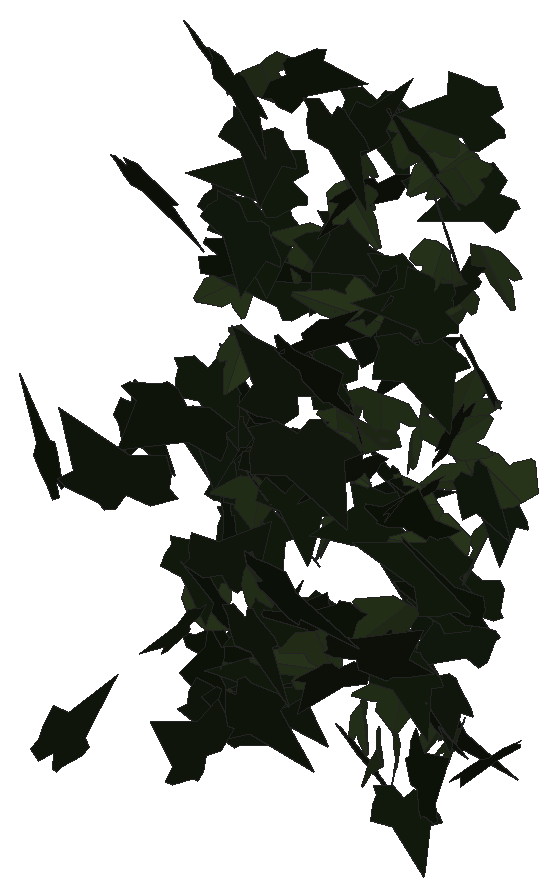
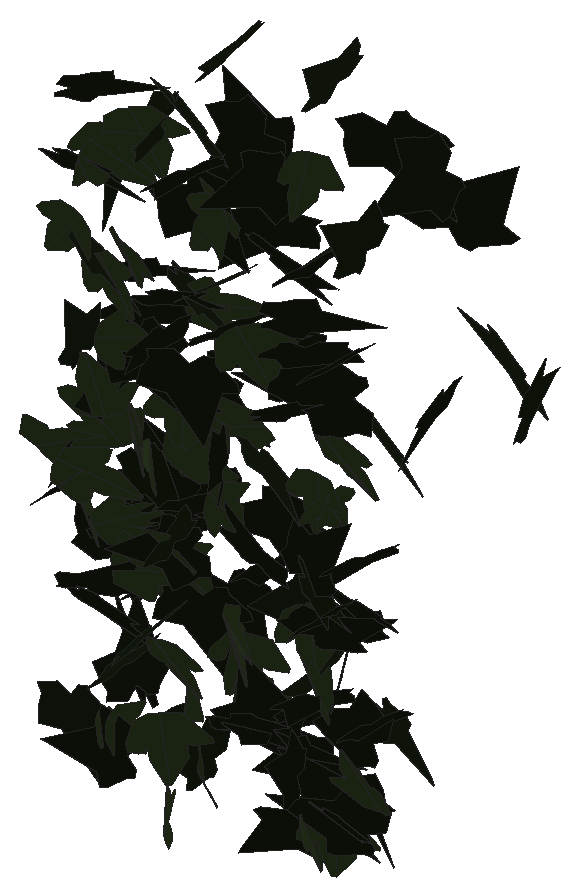
# SketchUp Ruby script. Lengths in inches.
U = 1.inch
M = Sketchup.active_model
def pt(a) = Geom::Point3d.new(a.map { |v| v * U })
def face(e, loops, mat)
  f = e.add_face(loops[0].map { |a| pt(a) })
  loops[1..].each { |l| e.add_face(l.map { |a| pt(a) }).erase! }
  f.material = f.back_material = mat if mat
  f
end
# faces: each face lists its corners as indices into pts; further lists are holes
def faces(e, pts, list, mat = nil) = list.each { |f| face(e, (f[0].is_a?(Array) ? f : [f]).map { |l| l.map { |i| pts[i] } }, mat) }
# xy, xz, yz: faces in a plane at the given z, y or x. An outline is a flat list of corners, or four numbers for a rectangle; further outlines are holes
def ring(l) = l.size == 4 ? [[l[0], l[1]], [l[2], l[1]], [l[2], l[3]], [l[0], l[3]]] : l.each_slice(2).to_a
def flat(e, list, mat, &to3) = list.each { |f| face(e, (f[0].is_a?(Array) ? f : [f]).map { |l| ring(l).map { |u, v| to3.(u, v) } }, mat) }
def xy(e, z, list, mat = nil) = flat(e, list, mat) { |x, y| [x, y, z] }
def xz(e, y, list, mat = nil) = flat(e, list, mat) { |x, z| [x, y, z] }
def yz(e, x, list, mat = nil) = flat(e, list, mat) { |y, z| [x, y, z] }
def lines(e, pts, list) = list.each { |a, b| e.add_line(pt(pts[a]), pt(pts[b])) }
# prism: a flat outline (further loops are holes) pulled along v
def prism(e, loops, v, mat = nil)
  f = face(e, loops, mat); d = Geom::Vector3d.new(v.map { |x| x * U })
  f.pushpull(f.normal.samedirection?(d) ? d.length : -d.length)
end
def box(e, o, s, mat = nil) = prism(e, [[o, [o[0] + s[0], o[1], o[2]], [o[0] + s[0], o[1] + s[1], o[2]], [o[0], o[1] + s[1], o[2]]]], [0, 0, s[2]], mat)
def at(x, y, z, deg = 0) = Geom::Transformation.translation(pt([x, y, z])) * Geom::Transformation.rotation(ORIGIN, Z_AXIS, deg.degrees)
def axes(o, x, y, z) = Geom::Transformation.new([*x, 0, *y, 0, *z, 0, *pt(o).to_a, 1])
def part(name) = M.definitions.add(name)
# library, detail: a bought-in or finely detailed component or shape, given as its bounding box
def library(name, o, s) = part(name).tap { |d| box(d.entities, o, s) }
def detail(e, o, s) = box(e.add_group.entities, o, s)
def put(e, d, t, mat = nil) = e.add_instance(d, t).tap { |i| i.material = mat if mat }
def group(e, t, mat = nil) = e.add_group.tap { |g| g.transformation = t; g.material = mat if mat }.entities
root = M.entities
M.materials.add("1026 AP 7946 SUNNY SIDE UP").color = [254, 231, 186]
M.materials.add("efeu1").color = [18, 25, 13]
M.materials.add("efeu2").color = [43, 57, 29]
c1 = part("ivyleaf_9")
p = [[1.54,2.16,1.25],[1.36,2.04,1.19],[-0.21,0.99,0.68],[-0.71,1.11,0.82],[-0.85,0.86,0.67],[-0.8,0.17,0.21],
  [-0.9,-0.01,0.1],[-0.67,-0.16,-0.02],[-0.08,-0.08,-0.05],[-0.03,-0.6,-0.4],[0.65,-0.88,-0.66],[0.83,-0.6,-0.49],
  [1.29,-0.42,-0.43],[1.8125,-0.07,-0.26],[1.21,0.44,0.15]]
faces(c1.entities,p,[[0,1,2,3,4,5,6,7,8,9,10,11,12,13,14]],"efeu1")
c2 = part("ivyleaf_10")
p = [[0,0.5,-0.03],[-0.0625,2.02,-0.43],[-0.19,2.01,-0.46],[-0.54,1.05,-0.29],[-0.52,0.625,-0.18],[-0.83,0.76,-0.28],
  [-1.16,0.64,-0.33],[-1.15,0.33,-0.24],[-0.77,-0.39,0.02],[-0.3,-0.51,0.16],[0.04,-0.48,0.23],[-0.02,2.01,-0.4375],
  [-0.06,2.01,-0.43],[0.04,-0.49,0.23],[0.67,-0.49,0.14],[1.38,0.36,-0.2],[1.375,0.51,-0.24],[0.81,0.65,-0.19],
  [0.62,0.59,-0.15],[0.6,1.09,-0.28],[0.5,1.23,-0.31]]
faces(c2.entities,p,[[0,1,2,3,4,5,6,7,8,9,10],[11,12,0,13,14,15,16,17,18,19,20]],"efeu2")
put(root,c1,axes([131.6,211.27,289.91],[0.23518,-0.30106,0.23677],[0.13886,-0.21446,-0.34729],[0.58083,0.17317,-0.01284]),"1026 AP 7946 SUNNY SIDE UP")
put(root,c2,axes([131.79,210.89,280.6],[0.50746,-0.14777,-0.11844],[0.18548,-0.01531,0.36395],[-0.22758,-0.34198,0.03251]),"1026 AP 7946 SUNNY SIDE UP")
put(root,c1,axes([131.84,211,284.61],[0.01812,-0.35592,-0.09361],[0.04573,0.0895,-0.36494],[0.57501,0.0041,0.03198]),"1026 AP 7946 SUNNY SIDE UP")
put(root,c2,axes([132.27,211.07,286.31],[0.41275,-0.15958,-0.19662],[-0.28987,0.0596,-0.31368],[0.26106,0.31849,-0.03742]),"1026 AP 7946 SUNNY SIDE UP")
put(root,c1,axes([132.3125,206.69,284.91],[-0.05121,-0.31432,0.36627],[0.04505,0.35621,0.32758],[-0.74694,0.04304,-0.00535]),"1026 AP 7946 SUNNY SIDE UP")
put(root,c1,axes([131.97,210.61,281.66],[-0.06706,-0.33394,-0.00524],[0.00686,0.00266,-0.34677],[0.52506,-0.04268,0.00386]),"1026 AP 7946 SUNNY SIDE UP")
put(root,c1,axes([132.09,210.98,283.83],[-0.36705,-0.1455,-0.19681],[0.34263,-0.01885,-0.26074],[0.15621,-0.30053,0.10946]),"1026 AP 7946 SUNNY SIDE UP")
put(root,c1,axes([132.59,209.53,281.15],[-0.289,0.28103,-0.06255],[0.03059,-0.06164,-0.34584],[-0.45159,-0.18402,0.01661]),"1026 AP 7946 SUNNY SIDE UP")
put(root,c1,axes([132.76,210.9,282.99],[-0.02142,0.10986,0.3543],[-0.56351,0.03263,-0.02522],[-0.06064,-0.34201,0.10918]),"1026 AP 7946 SUNNY SIDE UP")
put(root,c1,axes([132.35,211.45,283.59],[-0.11878,-0.29894,0.12842],[-0.03821,-0.12416,-0.31831],[0.50889,-0.0791,0.00607]),"1026 AP 7946 SUNNY SIDE UP")
put(root,c1,axes([132.6,210.87,280.07],[-0.50815,0.01624,-0.07065],[0.10517,-0.03216,-0.33227],[-0.03538,-0.32882,0.02706]),"1026 AP 7946 SUNNY SIDE UP")
put(root,c1,axes([132.87,209.92,280.27],[-0.02729,-0.04623,-0.47909],[-0.70907,0.12283,0.00548],[0.19134,0.44859,-0.04802]),"1026 AP 7946 SUNNY SIDE UP")
put(root,c2,axes([132.5625,210.75,279.8],[-0.50716,-0.11392,0.02457],[-0.01975,-0.0377,-0.35114],[0.18215,-0.32126,0.03035]),"1026 AP 7946 SUNNY SIDE UP")
put(root,c1,axes([132.05,210.74,279.91],[0.22263,-0.00495,0.34114],[0.50549,-0.08462,-0.14339],[0.12533,0.35009,-0.02766]),"1026 AP 7946 SUNNY SIDE UP")
put(root,c2,axes([132.53,210.94,285.28],[0.19134,0.2721,-0.16655],[-0.10349,-0.14936,-0.30794],[-0.48806,0.13835,0]),"1026 AP 7946 SUNNY SIDE UP")
put(root,c1,axes([132.4,211.04,287.62],[-0.09066,-0.35275,0.09344],[0.00197,-0.09405,-0.36841],[0.57349,-0.05544,0.01604]),"1026 AP 7946 SUNNY SIDE UP")
put(root,c1,axes([132.35,210.89,282.35],[0.12253,-0.14982,-0.33543],[0.42233,-0.19494,0.15791],[-0.37132,-0.27116,0.06892]),"1026 AP 7946 SUNNY SIDE UP")
put(root,c1,axes([132.71,211.16,284.02],[-0.39831,0.15679,-0.237],[0.25972,-0.16721,-0.30457],[-0.35382,-0.29924,0.04323]),"1026 AP 7946 SUNNY SIDE UP")
put(root,c2,axes([132.3125,211.27,282.1875],[-0.14424,0.08858,0.36734],[0.48412,-0.18108,0.12706],[0.31386,0.32002,-0.02717]),"1026 AP 7946 SUNNY SIDE UP")
put(root,c1,axes([132.18,210.41,281.21],[0.30764,-0.16116,0.29548],[0.29656,-0.21976,-0.26021],[0.42539,0.26976,-0.03228]),"1026 AP 7946 SUNNY SIDE UP")
put(root,c1,axes([132.88,211.03,284.05],[0.19162,-0.24095,0.31287],[-0.19767,0.2781,0.27965],[-0.57843,-0.17486,0.00808]),"1026 AP 7946 SUNNY SIDE UP")
put(root,c2,axes([132.78,210.92,285.45],[-0.49241,0.12376,0.05803],[-0.106,-0.02049,-0.34414],[-0.18515,-0.3174,0.04269]),"1026 AP 7946 SUNNY SIDE UP")
put(root,c1,axes([132.5,211.26,282.2],[-0.0606,-0.32371,-0.13287],[0.07923,0.12137,-0.33338],[0.54108,-0.05403,0.03394]),"1026 AP 7946 SUNNY SIDE UP")
put(root,c1,axes([133.14,211.27,288.23],[-0.37173,-0.04146,0.31601],[-0.45676,-0.10446,-0.2456],[0.16918,-0.37312,0.03127]),"1026 AP 7946 SUNNY SIDE UP")
put(root,c1,axes([132.74,208.0625,285.64],[0.2653,-0.27028,-0.29949],[-0.28404,0.22713,-0.32595],[0.5538,0.24597,-0.02371]),"1026 AP 7946 SUNNY SIDE UP")
put(root,c1,axes([132.37,210.67,286.93],[0.26777,0.141,-0.36208],[0.36476,0.26686,0.22713],[0.47214,-0.28614,0.02987]),"1026 AP 7946 SUNNY SIDE UP")
put(root,c2,axes([132.97,210.8125,283.14],[-0.37341,-0.31154,0.02105],[0.00818,-0.03183,-0.40302],[0.49104,-0.23638,0.02272]),"1026 AP 7946 SUNNY SIDE UP")
put(root,c1,axes([132.59,208.26,289.51],[0.65435,-0.13836,-0.02445],[-0.05367,-0.03021,-0.45014],[0.2139,0.41569,-0.03814]),"1026 AP 7946 SUNNY SIDE UP")
put(root,c2,axes([132.98,210.83,279.77],[0.07738,-0.32768,-0.00258],[-0.00809,-0.00012,-0.34132],[0.51518,0.04922,-0.00497]),"1026 AP 7946 SUNNY SIDE UP")
put(root,c1,axes([132.875,210.98,289.07],[-0.08575,-0.36419,0.0644],[-0.01008,-0.06434,-0.37973],[0.58151,-0.05482,0.00291]),"1026 AP 7946 SUNNY SIDE UP")
put(root,c1,axes([132.91,210.96,287.67],[-0.27093,-0.3178,-0.13334],[0.10467,0.10906,-0.37172],[0.52822,-0.18461,0.00527]),"1026 AP 7946 SUNNY SIDE UP")
put(root,c1,axes([133.45,211.18,286.49],[-0.32267,0.00841,0.28239],[-0.36237,-0.19076,-0.17285],[0.2336,-0.28431,0.12192]),"1026 AP 7946 SUNNY SIDE UP")
put(root,c2,axes([133.16,210.62,290.44],[-0.21397,-0.32823,-0.16326],[0.1082,0.14096,-0.36511],[0.56152,-0.15223,0.00814]),"1026 AP 7946 SUNNY SIDE UP")
put(root,c1,axes([133.16,210.88,280.51],[0.00995,-0.00698,0.37489],[0.23317,0.33248,0.00585],[-0.52272,0.14818,0.00975]),"1026 AP 7946 SUNNY SIDE UP")
put(root,c1,axes([133.09,210.84,279.7],[-0.0747,-0.10461,-0.32105],[0.27179,0.25918,-0.11548],[0.43862,-0.17841,0.01688]),"1026 AP 7946 SUNNY SIDE UP")
put(root,c1,axes([133.08,209.8,279.53],[-0.20685,0.00434,0.38335],[0.57991,-0.05099,0.13464],[0.07785,0.39135,0.01562]),"1026 AP 7946 SUNNY SIDE UP")
put(root,c1,axes([133.23,209.62,282.27],[-0.28347,0.00279,0.3015],[0.45966,0.01806,0.18545],[-0.02187,0.34325,-0.01019]),"1026 AP 7946 SUNNY SIDE UP")
put(root,c1,axes([133.63,210.63,281.16],[-0.29612,-0.17891,0.22532],[-0.22291,-0.16895,-0.26788],[0.38578,-0.23495,0.01817]),"1026 AP 7946 SUNNY SIDE UP")
put(root,c1,axes([133.09,210.58,283.33],[0.43914,-0.29736,0.11116],[0.07997,-0.10213,-0.41959],[0.49186,0.28209,-0.03103]),"1026 AP 7946 SUNNY SIDE UP")
put(root,c1,axes([133.89,210.78,285.48],[-0.18555,0.3047,0.10413],[-0.09166,0.0837,-0.33529],[-0.49553,-0.12957,0.02303]),"1026 AP 7946 SUNNY SIDE UP")
put(root,c1,axes([133.47,210.91,290.3125],[0.04861,0.09237,-0.3895],[-0.07452,0.37787,0.0932],[0.60824,0.03892,0.04254]),"1026 AP 7946 SUNNY SIDE UP")
put(root,c1,axes([134.07,210.27,280.5],[-0.41298,0.03013,0.21787],[-0.33558,-0.03081,-0.26891],[-0.00627,-0.33569,0.04225]),"1026 AP 7946 SUNNY SIDE UP")
put(root,c2,axes([133.89,211.16,287.54],[-0.35975,-0.27341,0.16517],[-0.08192,-0.1645,-0.36304],[0.49285,-0.22691,0.06022]),"1026 AP 7946 SUNNY SIDE UP")
put(root,c1,axes([133.66,209.63,288.39],[-0.08924,-0.38392,0.16398],[0.00226,-0.16302,-0.40005],[0.65483,-0.05176,0.02373]),"1026 AP 7946 SUNNY SIDE UP")
put(root,c1,axes([133.46,209.72,280.15],[-0.04871,-0.07153,-0.40567],[0.53191,0.20563,-0.06476],[0.33513,-0.33677,0.04382]),"1026 AP 7946 SUNNY SIDE UP")
put(root,c1,axes([133.625,209.69,281.53],[0.26264,-0.3687,-0.00189],[-0.01635,-0.00499,-0.41685],[0.57951,0.16696,-0.0109]),"1026 AP 7946 SUNNY SIDE UP")
put(root,c1,axes([133.76,210.7,281.04],[0.48558,0.15081,0.09062],[-0.14355,-0.01083,0.35269],[0.23321,-0.32068,0.02841]),"1026 AP 7946 SUNNY SIDE UP")
put(root,c1,axes([133.96,210.8,283.75],[-0.39278,0.21861,0.17515],[0.16973,-0.1322,0.3402],[0.39972,0.27094,0.02766]),"1026 AP 7946 SUNNY SIDE UP")
put(root,c2,axes([134.08,211.23,282.76],[0.21848,-0.35344,-0.05587],[-0.03386,0.04765,-0.39095],[0.56076,0.14058,-0.00184]),"1026 AP 7946 SUNNY SIDE UP")
put(root,c1,axes([134.17,211.05,281.15],[-0.44348,-0.1535,0.04482],[-0.04177,-0.04374,-0.33002],[0.24776,-0.28214,0.0246]),"1026 AP 7946 SUNNY SIDE UP")
put(root,c1,axes([133.72,209.28,291.06],[0.17773,-0.37057,0.18777],[0.07105,-0.17894,-0.40009],[0.64694,0.12146,-0.00764]),"1026 AP 7946 SUNNY SIDE UP")
put(root,c1,axes([133.62,210.18,284.25],[0.21429,0.03441,-0.37262],[0.28073,0.33033,0.10355],[0.49792,-0.20105,0.10198]),"1026 AP 7946 SUNNY SIDE UP")
put(root,c2,axes([134.08,211.21,282.82],[0.24089,-0.28966,0.10366],[0.04101,-0.1016,-0.33731],[0.48126,0.15364,-0.02314]),"1026 AP 7946 SUNNY SIDE UP")
put(root,c2,axes([133.76,209.56,282.45],[0.01423,0.00784,0.35575],[0.47375,-0.16901,-0.00517],[0.26545,0.30122,-0.00984]),"1026 AP 7946 SUNNY SIDE UP")
put(root,c1,axes([133.94,210.49,283.59],[-0.05928,-0.36956,-0.02782],[0.01156,0.02429,-0.38252],[0.58229,-0.0381,0.00476]),"1026 AP 7946 SUNNY SIDE UP")
put(root,c2,axes([134.62,210.08,280.91],[-0.04739,0.02263,0.35276],[-0.43255,-0.20688,-0.01207],[0.32226,-0.27436,0.03567]),"1026 AP 7946 SUNNY SIDE UP")
put(root,c2,axes([134.36,211.17,284.73],[-0.05619,-0.28349,0.21537],[0.05152,-0.21349,-0.29149],[0.55297,-0.00892,0.04905]),"1026 AP 7946 SUNNY SIDE UP")
put(root,c1,axes([134.46,211.05,287.47],[-0.27821,-0.31044,0.16465],[-0.06127,-0.16247,-0.36645],[0.54688,-0.17613,0.04271]),"1026 AP 7946 SUNNY SIDE UP")
put(root,c2,axes([134.52,211.07,289.32],[-0.4156,0.25016,-0.16252],[0.1526,-0.12851,-0.37482],[-0.44055,-0.2805,0.02349]),"1026 AP 7946 SUNNY SIDE UP")
put(root,c1,axes([135.04,204.96,286.35],[0.31632,0.0576,0.42442],[-0.64661,0.0943,0.19398],[-0.09535,-0.44837,0.09254]),"1026 AP 7946 SUNNY SIDE UP")
put(root,c1,axes([134.46,210.99,285.16],[0.19695,-0.14655,-0.38091],[0.55186,-0.13986,0.17918],[-0.29163,-0.36363,0.08181]),"1026 AP 7946 SUNNY SIDE UP")
put(root,c1,axes([134.92,210.9,287.89],[-0.32741,-0.1793,0.26976],[-0.11912,-0.27719,-0.25821],[0.48595,-0.18875,0.11846]),"1026 AP 7946 SUNNY SIDE UP")
put(root,c2,axes([134.86,209.875,281.6],[-0.3833,-0.25271,-0.10663],[0.14196,0.05434,-0.36039],[0.40435,-0.25863,0.02545]),"1026 AP 7946 SUNNY SIDE UP")
put(root,c1,axes([135.1,210.92,286.59],[0.32151,0.21894,-0.21709],[-0.20763,-0.16641,-0.30926],[-0.43186,0.243,-0.01294]),"1026 AP 7946 SUNNY SIDE UP")
put(root,c1,axes([135.3,209.79,286.17],[-0.22621,0.02611,0.3294],[-0.43333,-0.18916,-0.11298],[0.25779,-0.29506,0.09913]),"1026 AP 7946 SUNNY SIDE UP")
put(root,c1,axes([134.81,211.33,290.1],[0.02803,-0.39,-0.09193],[0.03859,0.08801,-0.40066],[0.62713,0.01202,0.02877]),"1026 AP 7946 SUNNY SIDE UP")
put(root,c2,axes([135.43,210.21,287.1875],[0.0801,0.07824,0.37855],[-0.46393,-0.22051,0.08933],[0.36461,-0.29777,0.0305]),"1026 AP 7946 SUNNY SIDE UP")
put(root,c2,axes([134.81,210.89,279.85],[0.17007,-0.06052,0.32689],[0.37178,-0.21369,-0.12613],[0.34685,0.25872,-0.02508]),"1026 AP 7946 SUNNY SIDE UP")
put(root,c2,axes([135.33,210.59,284.8],[-0.44218,-0.07847,-0.19529],[-0.25243,-0.11492,0.29438],[-0.19983,0.31881,0.06027]),"1026 AP 7946 SUNNY SIDE UP")
put(root,c1,axes([135.39,210.55,289.25],[-0.12575,0.32024,-0.28768],[0.04827,-0.28091,-0.34035],[-0.66824,-0.08055,0.02956]),"1026 AP 7946 SUNNY SIDE UP")
put(root,c1,axes([135.79,208.09,286.91],[-0.54226,-0.005,-0.26372],[-0.40147,0.03809,0.35385],[0.02941,0.42777,-0.03207]),"1026 AP 7946 SUNNY SIDE UP")
put(root,c1,axes([135.1,210.91,283.6],[0.09248,0.20089,-0.28899],[0.02034,0.28422,0.21328],[0.54361,-0.04481,0.04119]),"1026 AP 7946 SUNNY SIDE UP")
put(root,c2,axes([134.99,210.4,289.03],[0.35423,-0.02648,0.31422],[0.4651,-0.07962,-0.23254],[0.12514,0.37086,-0.02521]),"1026 AP 7946 SUNNY SIDE UP")
put(root,c2,axes([135.17,211.32,279.18],[-0.09734,0.07694,0.3774],[0.37137,-0.27948,0.10007],[0.45579,0.24414,-0.00094]),"1026 AP 7946 SUNNY SIDE UP")
put(root,c1,axes([135.08,211.33,283.89],[0.18878,-0.29851,0.1501],[0.10903,-0.13083,-0.33191],[0.512,0.13793,0.01534]),"1026 AP 7946 SUNNY SIDE UP")
put(root,c1,axes([135.28,210.35,290.12],[-0.22555,0.35026,0.10424],[0.08439,-0.08511,0.38904],[0.56616,0.15222,-0.01646]),"1026 AP 7946 SUNNY SIDE UP")
put(root,c1,axes([135.68,210.37,287.59],[-0.44235,0.23956,-0.08108],[0.05875,-0.07906,-0.37939],[-0.39279,-0.28161,0.03457]),"1026 AP 7946 SUNNY SIDE UP")
put(root,c2,axes([135.02,209.6,285.08],[0.2355,0.09834,0.31005],[0.44402,0.10775,-0.18074],[-0.22334,0.31791,-0.0324]),"1026 AP 7946 SUNNY SIDE UP")
put(root,c2,axes([135.79,211.23,283.61],[-0.25763,0.03177,0.29292],[-0.38668,-0.18273,-0.1261],[0.22936,-0.27239,0.11643]),"1026 AP 7946 SUNNY SIDE UP")
put(root,c1,axes([135.32,203,282.87],[-0.25924,0.43642,0.11952],[0.07277,-0.10387,0.47995],[0.70532,0.17112,-0.00559]),"1026 AP 7946 SUNNY SIDE UP")
put(root,c1,axes([135.58,210,282.2],[0.28588,0.20905,-0.23074],[-0.18833,-0.19272,-0.28508],[-0.4449,0.21591,-0.02759]),"1026 AP 7946 SUNNY SIDE UP")
put(root,c2,axes([135.5625,210.97,280.49],[-0.38885,-0.31016,0.03031],[-0.00123,-0.03918,-0.40815],[0.49015,-0.24615,0.02302]),"1026 AP 7946 SUNNY SIDE UP")
put(root,c2,axes([135.58,210.51,285.61],[-0.53609,-0.04863,0.03153],[-0.03989,-0.03969,-0.35312],[0.08132,-0.34003,0.03465]),"1026 AP 7946 SUNNY SIDE UP")
put(root,c1,axes([135.8125,205.4375,287.84],[0.24991,0.10689,-0.42343],[-0.45155,-0.29715,-0.19546],[-0.49323,0.32619,-0.0356]),"1026 AP 7946 SUNNY SIDE UP")
put(root,c1,axes([135.74,210.9,287.52],[-0.44666,-0.12502,0.16117],[-0.17349,-0.1303,-0.31301],[0.26384,-0.29734,0.06702]),"1026 AP 7946 SUNNY SIDE UP")
put(root,c2,axes([135.72,210.68,281.6],[0.45851,-0.14146,-0.12798],[-0.20172,0.01634,-0.33141],[0.21553,0.31622,-0.03791]),"1026 AP 7946 SUNNY SIDE UP")
put(root,c1,axes([135.87,210.37,283.68],[-0.34939,-0.11597,0.29358],[-0.32952,-0.20141,-0.25337],[0.35551,-0.30066,0.05368]),"1026 AP 7946 SUNNY SIDE UP")
put(root,c1,axes([135.27,210.2,279.77],[0.34505,-0.27164,0.12006],[0.09595,-0.10235,-0.35997],[0.45575,0.22721,-0.01512]),"1026 AP 7946 SUNNY SIDE UP")
put(root,c2,axes([136.13,210.95,282.9375],[-0.01716,-0.02669,-0.40695],[-0.58067,-0.14138,0.01954],[-0.22381,0.36885,-0.01947]),"1026 AP 7946 SUNNY SIDE UP")
put(root,c1,axes([135.94,209.49,285.19],[-0.15122,0.16307,-0.30651],[0.05188,-0.30422,-0.18397],[-0.53224,-0.07599,0.06915]),"1026 AP 7946 SUNNY SIDE UP")
put(root,c1,axes([135.93,208.96,281.82],[0.00767,0.27342,-0.22868],[-0.00978,-0.22345,-0.28302],[-0.55523,0.00771,0.00182]),"1026 AP 7946 SUNNY SIDE UP")
put(root,c1,axes([135.62,210.88,286.96],[0.16021,-0.32721,-0.25123],[-0.14561,0.22429,-0.35126],[0.62315,0.13653,-0.01749]),"1026 AP 7946 SUNNY SIDE UP")
put(root,c1,axes([136.01,211.25,281.72],[-0.04062,-0.37619,0.0667],[0.00438,0.06685,0.38885],[-0.60078,0.02592,-0.00168]),"1026 AP 7946 SUNNY SIDE UP")
put(root,c1,axes([135.55,209.34,290.97],[0.17968,-0.41648,0.02887],[-0.00512,-0.0324,-0.44493],[0.65659,0.11372,-0.01137]),"1026 AP 7946 SUNNY SIDE UP")
put(root,c2,axes([135.92,211.16,285.51],[0.23384,-0.30665,-0.11919],[-0.03865,0.11435,-0.34938],[0.51294,0.14841,0.02801]),"1026 AP 7946 SUNNY SIDE UP")
put(root,c2,axes([136.1,210.9,290.26],[-0.47903,-0.16981,0.16032],[-0.19673,-0.09655,-0.3592],[0.30532,-0.32864,0.02009]),"1026 AP 7946 SUNNY SIDE UP")
put(root,c2,axes([135.74,211.09,284.78],[-0.14858,-0.01741,-0.3497],[0.12001,-0.34431,-0.00571],[-0.52064,-0.0744,0.09848]),"1026 AP 7946 SUNNY SIDE UP")
put(root,c1,axes([136.13,210.77,286.61],[-0.0688,0.32342,-0.26915],[0.0328,-0.26251,-0.33755],[-0.65474,-0.04714,0.01137]),"1026 AP 7946 SUNNY SIDE UP")
put(root,c1,axes([135.74,210.82,290.32],[0.4079,-0.32646,0.00204],[-0.02423,-0.01713,-0.42903],[0.5128,0.25887,-0.0219]),"1026 AP 7946 SUNNY SIDE UP")
put(root,c2,axes([136.13,209.61,280.21],[0.07353,-0.26596,-0.25437],[0.00144,0.24753,-0.27473],[0.56902,0.03374,0.03357]),"1026 AP 7946 SUNNY SIDE UP")
put(root,c2,axes([136.13,211.48,286.94],[0.00349,-0.09313,0.36325],[0.02375,-0.35282,-0.09802],[0.57377,0.01517,0.00185]),"1026 AP 7946 SUNNY SIDE UP")
put(root,c2,axes([136.29,209.91,282.54],[-0.19577,-0.25821,0.25662],[-0.15118,-0.23163,-0.29647],[0.54517,-0.15695,0.00994]),"1026 AP 7946 SUNNY SIDE UP")
put(root,c1,axes([136.32,210.39,284.38],[-0.14792,0.30868,-0.1584],[0.06473,-0.15001,-0.33329],[-0.53961,-0.10261,0.00344]),"1026 AP 7946 SUNNY SIDE UP")
put(root,c2,axes([136.42,211.2,289.81],[-0.28749,-0.19792,0.30916],[-0.14865,-0.2996,-0.26367],[0.54689,-0.18548,0.09085]),"1026 AP 7946 SUNNY SIDE UP")
put(root,c1,axes([136.6,210.6,287.51],[-0.36901,-0.00916,0.27299],[-0.36833,-0.15877,-0.22026],[0.19551,-0.31641,0.1003]),"1026 AP 7946 SUNNY SIDE UP")
put(root,c2,axes([136.58,211.06,287.78],[-0.38233,0.08012,0.24718],[-0.38255,0.01477,-0.25948],[-0.10641,-0.34096,0.04473]),"1026 AP 7946 SUNNY SIDE UP")
put(root,c1,axes([136.72,204.77,282.51],[-0.24689,0.3508,0.28466],[-0.20399,0.24223,-0.39419],[-0.66986,-0.20306,0.01512]),"1026 AP 7946 SUNNY SIDE UP")
put(root,c2,axes([136.23,210.96,288.17],[0.44756,-0.19372,0.06396],[0.05689,-0.05878,-0.35389],[0.31531,0.28558,-0.02694]),"1026 AP 7946 SUNNY SIDE UP")
put(root,c1,axes([136.15,210.3,283.8],[0.5201,0.04992,0.10861],[-0.17068,0.01794,0.3431],[0.06607,-0.34662,0.03133]),"1026 AP 7946 SUNNY SIDE UP")
put(root,c2,axes([136.35,210.98,280.26],[-0.00691,-0.26417,0.25553],[0.06204,-0.24843,-0.27167],[0.56802,0.02392,0.03278]),"1026 AP 7946 SUNNY SIDE UP")
put(root,c2,axes([136.68,210.73,283.375],[0.05799,0.12508,0.36875],[-0.21342,-0.33069,0.13178],[0.55557,-0.14009,0.01213]),"1026 AP 7946 SUNNY SIDE UP")
put(root,c2,axes([136.875,211.34,284.48],[-0.18234,-0.08288,0.36142],[-0.37628,-0.25858,-0.14573],[0.42488,-0.26457,0.02604]),"1026 AP 7946 SUNNY SIDE UP")
put(root,c1,axes([136.08,211.21,279.99],[0.41777,-0.14629,0.22185],[0.27128,-0.13306,-0.31198],[0.308,0.31562,-0.02613]),"1026 AP 7946 SUNNY SIDE UP")
put(root,c1,axes([136.38,210.34,286.88],[-0.12047,-0.33594,-0.21556],[0.08635,0.20008,-0.35371],[0.61471,-0.09394,0.00744]),"1026 AP 7946 SUNNY SIDE UP")
put(root,c2,axes([136.5625,211.14,285.59],[-0.33608,-0.27905,0.04968],[0.02353,0.05119,0.36188],[-0.44509,0.21341,-0.01838]),"1026 AP 7946 SUNNY SIDE UP")
put(root,c2,axes([136.67,210.89,280.16],[0.04611,-0.32238,-0.04196],[-0.00784,0.03861,-0.33325],[0.51053,0.02971,-0.00132]),"1026 AP 7946 SUNNY SIDE UP")
put(root,c1,axes([136.95,211.24,290.69],[-0.36565,-0.05212,0.29013],[-0.3817,-0.15736,-0.23716],[0.23987,-0.32984,0.06488]),"1026 AP 7946 SUNNY SIDE UP")
put(root,c2,axes([136.46,210.97,285.05],[-0.38914,-0.15283,0.20909],[0.23846,0.13995,0.29862],[-0.32188,0.28845,-0.03155]),"1026 AP 7946 SUNNY SIDE UP")
put(root,c1,axes([136.93,210.92,282.34],[-0.52294,-0.19551,0.05939],[0.05612,0.0549,0.39664],[-0.31606,0.33323,-0.02783]),"1026 AP 7946 SUNNY SIDE UP")
put(root,c1,axes([136.54,207.47,288.38],[0.26736,0.308,0.26163],[0.23542,0.20464,-0.36024],[-0.58,0.22504,-0.02562]),"1026 AP 7946 SUNNY SIDE UP")
put(root,c1,axes([136.93,211.01,288.02],[-0.35728,0.26426,-0.04823],[0.02234,-0.05137,-0.35859],[-0.42183,-0.22655,0.02186]),"1026 AP 7946 SUNNY SIDE UP")
put(root,c1,axes([137,210.42,283.17],[-0.17542,-0.35958,-0.22247],[-0.08418,-0.2073,0.38654],[-0.65248,0.12342,0.00995]),"1026 AP 7946 SUNNY SIDE UP")
put(root,c1,axes([136.48,210.72,281.1],[0.01253,-0.37174,0.14512],[0.03904,-0.14227,-0.38331],[0.62505,0.01634,0.02103]),"1026 AP 7946 SUNNY SIDE UP")
put(root,c1,axes([136.89,210.35,282.63],[0.39455,-0.10913,0.30472],[-0.39262,0.1633,0.28066],[-0.30416,-0.35235,0.03299]),"1026 AP 7946 SUNNY SIDE UP")
put(root,c1,axes([137.02,210.875,282.13],[-0.61942,0.03811,-0.01755],[0.02101,-0.04021,-0.406],[-0.06234,-0.39225,0.03757]),"1026 AP 7946 SUNNY SIDE UP")
put(root,c1,axes([136.53,210.33,280.65],[0.54742,-0.23981,-0.08849],[0.14314,-0.01629,0.43369],[-0.37332,-0.35789,0.03652]),"1026 AP 7946 SUNNY SIDE UP")
put(root,c1,axes([136.77,210.45,285.33],[0.0777,0.11414,0.41172],[0.24184,0.36818,-0.12597],[-0.6061,0.16154,0.00252]),"1026 AP 7946 SUNNY SIDE UP")
put(root,c2,axes([136.74,210.87,289.78],[-0.24425,-0.30073,-0.17511],[0.19986,0.12157,-0.34398],[0.50366,-0.19408,0.05158]),"1026 AP 7946 SUNNY SIDE UP")
put(root,c1,axes([137.17,211.2,289.45],[-0.54427,0.00019,0.07228],[-0.10952,-0.04367,-0.3541],[0.01335,-0.35047,0.04208]),"1026 AP 7946 SUNNY SIDE UP")
put(root,c1,axes([136.91,210.26,289.31],[0.37486,-0.13645,-0.32653],[-0.46849,0.11112,-0.28017],[0.27153,0.38008,-0.03261]),"1026 AP 7946 SUNNY SIDE UP")
put(root,c1,axes([136.63,207.18,286.84],[-0.17195,-0.31156,-0.31381],[0.19891,0.27593,-0.33788],[0.65359,-0.16594,0.02027]),"1026 AP 7946 SUNNY SIDE UP")
put(root,c1,axes([136.32,206.82,284.39],[0.43254,-0.18349,0.31729],[0.35407,-0.21532,-0.33946],[0.44046,0.35328,-0.03871]),"1026 AP 7946 SUNNY SIDE UP")
put(root,c1,axes([136.7,209.6,281.9375],[0.02364,-0.36698,-0.05226],[0.0229,0.04923,-0.37771],[0.58163,0.01298,0.017]),"1026 AP 7946 SUNNY SIDE UP")
put(root,c1,axes([136.77,209.53,279.62],[0.00148,-0.34413,-0.06665],[-0.00047,0.06275,-0.35416],[0.55004,0.00098,-0.00012]),"1026 AP 7946 SUNNY SIDE UP")
put(root,c1,axes([136.61,207.27,287.94],[0.61284,-0.12457,-0.16693],[0.27331,0.02131,0.41577],[-0.16739,-0.42128,0.0677]),"1026 AP 7946 SUNNY SIDE UP")
put(root,c1,axes([136.9,211.14,286.39],[0.05494,-0.19586,0.31627],[0.09532,-0.30211,-0.20669],[0.5661,0.06988,0.00411]),"1026 AP 7946 SUNNY SIDE UP")
put(root,c1,axes([136.82,208.4,282.58],[0.6284,0.17718,-0.0133],[-0.0084,0.04623,0.4483],[0.27932,-0.3972,0.04342]),"1026 AP 7946 SUNNY SIDE UP")
put(root,c2,axes([137.5,211.12,284.53],[0.37659,0.11917,0.29141],[-0.43439,-0.07074,0.27191],[0.20811,-0.3633,0.04021]),"1026 AP 7946 SUNNY SIDE UP")
put(root,c2,axes([137.25,210.72,283.69],[0.23254,-0.35241,-0.01758],[-0.02035,0.0109,-0.39358],[0.55426,0.14825,-0.00707]),"1026 AP 7946 SUNNY SIDE UP")
put(root,c1,axes([137.11,210.76,284.72],[0.17308,-0.25245,-0.22577],[-0.1681,0.19044,-0.28205],[0.4965,0.15248,-0.01679]),"1026 AP 7946 SUNNY SIDE UP")
put(root,c2,axes([137.11,211.12,288.36],[-0.44996,0.13491,-0.15611],[0.18253,-0.1076,-0.32351],[-0.26274,-0.30579,0.0426]),"1026 AP 7946 SUNNY SIDE UP")
put(root,c1,axes([137.09,211.35,284.15],[-0.02929,-0.34203,0.07975],[-0.00725,-0.07922,-0.35335],[0.55205,-0.01919,-0.00041]),"1026 AP 7946 SUNNY SIDE UP")
put(root,c1,axes([137.51,210.61,280.14],[-0.05747,0.3756,-0.07111],[0.00474,-0.0712,-0.38916],[-0.60108,-0.03647,0.00373]),"1026 AP 7946 SUNNY SIDE UP")
put(root,c1,axes([137.1,209.47,279.99],[-0.08283,0.17798,0.43253],[0.10254,-0.41433,0.1874],[0.70819,0.08081,0.02346]),"1026 AP 7946 SUNNY SIDE UP")
